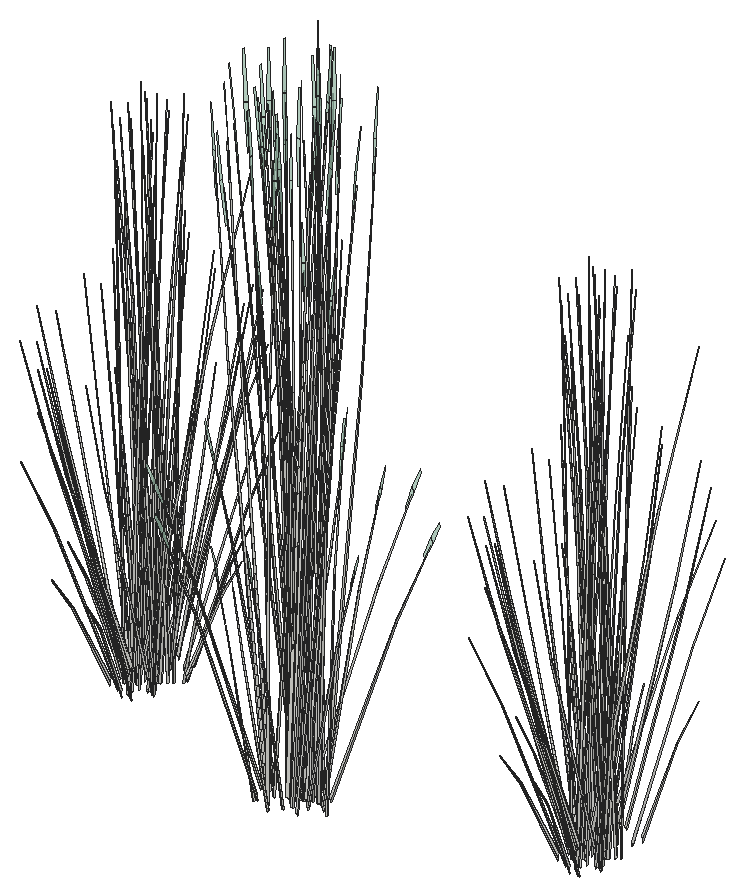
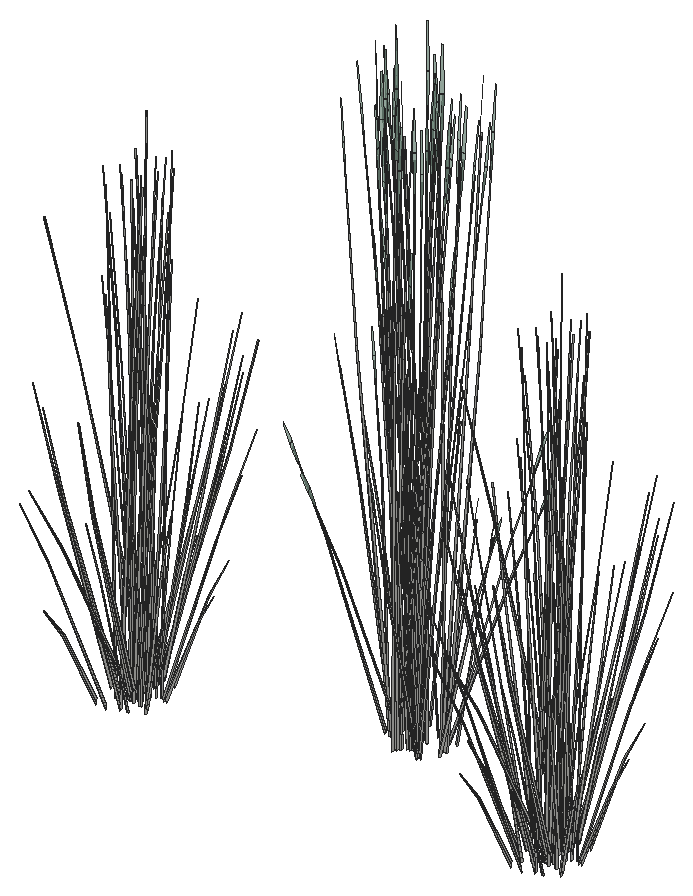
# SketchUp Ruby script. Lengths in inches.
U = 1.inch
M = Sketchup.active_model
def pt(a) = Geom::Point3d.new(a.map { |v| v * U })
def face(e, loops, mat)
  f = e.add_face(loops[0].map { |a| pt(a) })
  loops[1..].each { |l| e.add_face(l.map { |a| pt(a) }).erase! }
  f.material = f.back_material = mat if mat
  f
end
# faces: each face lists its corners as indices into pts; further lists are holes
def faces(e, pts, list, mat = nil) = list.each { |f| face(e, (f[0].is_a?(Array) ? f : [f]).map { |l| l.map { |i| pts[i] } }, mat) }
# xy, xz, yz: faces in a plane at the given z, y or x. An outline is a flat list of corners, or four numbers for a rectangle; further outlines are holes
def ring(l) = l.size == 4 ? [[l[0], l[1]], [l[2], l[1]], [l[2], l[3]], [l[0], l[3]]] : l.each_slice(2).to_a
def flat(e, list, mat, &to3) = list.each { |f| face(e, (f[0].is_a?(Array) ? f : [f]).map { |l| ring(l).map { |u, v| to3.(u, v) } }, mat) }
def xy(e, z, list, mat = nil) = flat(e, list, mat) { |x, y| [x, y, z] }
def xz(e, y, list, mat = nil) = flat(e, list, mat) { |x, z| [x, y, z] }
def yz(e, x, list, mat = nil) = flat(e, list, mat) { |y, z| [x, y, z] }
def lines(e, pts, list) = list.each { |a, b| e.add_line(pt(pts[a]), pt(pts[b])) }
# prism: a flat outline (further loops are holes) pulled along v
def prism(e, loops, v, mat = nil)
  f = face(e, loops, mat); d = Geom::Vector3d.new(v.map { |x| x * U })
  f.pushpull(f.normal.samedirection?(d) ? d.length : -d.length)
end
def box(e, o, s, mat = nil) = prism(e, [[o, [o[0] + s[0], o[1], o[2]], [o[0] + s[0], o[1] + s[1], o[2]], [o[0], o[1] + s[1], o[2]]]], [0, 0, s[2]], mat)
def at(x, y, z, deg = 0) = Geom::Transformation.translation(pt([x, y, z])) * Geom::Transformation.rotation(ORIGIN, Z_AXIS, deg.degrees)
def axes(o, x, y, z) = Geom::Transformation.new([*x, 0, *y, 0, *z, 0, *pt(o).to_a, 1])
def part(name) = M.definitions.add(name)
# library, detail: a bought-in or finely detailed component or shape, given as its bounding box
def library(name, o, s) = part(name).tap { |d| box(d.entities, o, s) }
def detail(e, o, s) = box(e.add_group.entities, o, s)
def put(e, d, t, mat = nil) = e.add_instance(d, t).tap { |i| i.material = mat if mat }
def group(e, t, mat = nil) = e.add_group.tap { |g| g.transformation = t; g.material = mat if mat }.entities
root = M.entities
M.materials.add("LightPink_Translucent").color = [175, 214, 192]
M.materials["LightPink_Translucent"].alpha = 0.75
c1 = part("blade")
p = [[2.15,0.21,22],[0,0.17,0],[0.09,0.45,0],[2.18,0.31,22],[2.29,0.31,22],[0.38,0.45,0],
  [2.48,0.24,33],[2.49,0.24,33],[2.48,0.22,33]]
faces(c1.entities,p,[[0,1,2,3],[4,5,2,3],[6,3,4,7],[8,0,3,6]])
c2 = part("blade with seeds\#1")
put(c2.entities,c1,at(0,0,0))
c3 = part("seeds")
p = [[0.3,-0.1,1.38],[-0.01,-0.03,1.59],[-0.01,-0.03,0.03],[0.14,-0.07,-0.07],[0.29,-0.03,3],[0.15,0.01,3.11]]
faces(c3.entities,p,[[0,1,2,3],[1,0,4,5]],"LightPink_Translucent")
c4 = part("blade with seeds")
put(c4.entities,c1,at(0,0,0))
put(c4.entities,c3,axes([2.4,0.25,30.99],[1.5799,-0.05474,1.17369],[-0.12525,1.92788,0.29478],[-0.07173,-0.02425,1.56792]))
put(root,c2,axes([371.35,242.3,138.84],[0.07713,0.14131,1.17311],[-0.13499,0.4232,-0.25229],[-0.16789,-0.07845,0.50157]))
put(root,c2,axes([371.62,242.95,140.8],[-0.30983,0.23727,-0.58282],[-0.17267,-0.48842,0.07033],[-0.1497,0.05548,0.82446]))
put(root,c2,axes([371.21,244.49,138.84],[0.12465,0.0301,1.17311],[0.10435,0.44009,-0.25229],[-0.16111,0.10287,0.50157]))
put(root,c2,axes([371.92,241.96,140.8],[-0.35246,-0.01294,-0.58282],[0.02367,-0.54471,0.07033],[-0.14932,-0.05748,0.82446]))
put(root,c2,axes([370.74,242.82,138.99],[0.2222,-0.06377,0.94226],[-0.12306,0.35378,0.69231],[-0.11377,-0.03807,0.20754]))
put(root,c2,axes([371.56,243.125,140.56],[-0.09552,0.48869,-0.41919],[-0.3275,-0.16751,-0.3247],[-0.13186,0.04481,0.80208]))
put(root,c2,axes([371.81,242.07,140.56],[-0.25603,0.35588,-0.41919],[-0.22422,-0.37594,-0.3247],[-0.13008,-0.05415,0.80208]))
put(root,c2,axes([371.01,244.64,138.99],[0.13262,-0.25932,0.94226],[0.07972,0.37767,0.69231],[-0.10192,0.08081,0.20754]))
put(root,c2,axes([371.71,244.02,140.8],[-0.18418,0.4239,-0.58282],[-0.32274,-0.30126,0.07033],[-0.10997,0.15358,0.82446]))
put(root,c2,axes([371.72,244.21,140.56],[0.09058,0.49056,-0.41919],[-0.34303,0.08581,-0.3247],[-0.0983,0.13176,0.80208]))
put(root,c2,axes([372.4,241.33,140.56],[-0.34793,0.12771,-0.41919],[-0.06086,-0.48364,-0.3247],[-0.09345,-0.1386,0.80208]))
put(root,c2,axes([372.54,241.32,140.8],[-0.30066,-0.25968,-0.58282],[0.21367,-0.45504,0.07033],[-0.10893,-0.15505,0.82446]))
put(root,c2,axes([372.26,240.94,138.84],[-0.01129,0.1776,1.17311],[-0.30276,0.18194,-0.25229],[-0.08565,-0.21818,0.50157]))
put(root,c2,axes([371.7,240.74,138.99],[0.19397,0.16559,0.94226],[-0.26061,0.14233,0.69231],[-0.0653,-0.13676,0.20754]))
put(root,c2,axes([372.26,245.28,138.84],[0.10609,-0.09706,1.17311],[0.28837,0.22366,-0.25229],[-0.06892,0.22965,0.50157]))
put(root,c2,axes([372.16,244.88,140.8],[-0.00917,0.49695,-0.58282],[-0.38634,-0.03338,0.07033],[-0.04077,0.21053,0.82446]))
put(root,c2,axes([372.24,245.05,140.56],[0.25241,0.36098,-0.41919],[-0.26664,0.31614,-0.3247],[-0.0384,0.18341,0.80208]))
put(root,c2,axes([373.06,243.43,138.71],[0.18468,-0.56014,0.19741],[0.38374,0.26958,0.41019],[-0.08846,0,1.31701]))
put(root,c2,axes([372.58,245.86,138.99],[-0.02727,-0.31739,0.94226],[0.24024,0.20133,0.69231],[-0.03604,0.15684,0.20754]))
put(root,c2,axes([372.8,243.62,138.95],[0.02352,0.53984,0.36702],[-0.39046,0.04882,-0.17663],[-0.03957,-0.09664,1.17838]))
put(root,c2,axes([373.08,245.01,138.75],[0.38104,0,0.40731],[0,0.5562,0],[-0.08679,0,1.29208]))
put(root,c2,axes([372.94,243.63,138.65],[0.42608,-0.21614,0.37535],[0.14817,0.61757,0.14729],[-0.07829,-0.00755,1.30318]))
put(root,c2,axes([373.17,241.11,140.56],[-0.34661,-0.13468,-0.41919],[0.1188,-0.46175,-0.3247],[-0.03178,-0.18591,0.80208]))
put(root,c2,axes([371.96,242.1,138.75],[-0.19052,0.46527,0.40731],[-0.34163,-0.2781,0],[0.04339,-0.10597,1.29208]))
put(root,c2,axes([373.28,243.74,138.95],[0.34335,0.2412,0.36702],[-0.16524,0.50118,-0.17663],[-0.07915,0,1.17838]))
put(root,c2,axes([372.7,243.15,138.65],[0.3458,0.41219,0.37535],[-0.30525,0.4897,0.14729],[-0.03451,-0.09937,1.30318]))
put(root,c2,axes([372.13,243.87,138.75],[0.37869,0.14361,0.14473],[-0.10717,0.52552,0.28783],[-0.00184,-0.09078,1.3159]))
put(root,c2,axes([373.3,241.19,140.8],[-0.16829,-0.43684,-0.58282],[0.34641,-0.24345,0.07033],[-0.03935,-0.21107,0.82446]))
put(root,c2,axes([372.55,242.77,138.86],[-0.34006,-0.0959,0.11878],[0.05903,-0.46856,-0.33919],[0.03492,-0.08527,1.03975]))
put(root,c2,axes([372.64,242.97,138.95],[-0.31983,0.29864,0.36702],[-0.22522,-0.45236,-0.17663],[0.03957,-0.09664,1.17838]))
put(root,c2,axes([373.36,243.58,138.65],[0.08028,-0.62833,0.37535],[0.45342,0.12787,0.14729],[-0.04378,0.09182,1.30318]))
put(root,c2,axes([372.15,242.28,138.75],[0.10113,0.5342,0.14473],[-0.37638,0.13191,0.28783],[0.05484,-0.04764,1.3159]))
put(root,c2,axes([374.08,243.92,138.75],[-0.10113,-0.5342,0.14473],[0.37638,-0.13191,0.28783],[-0.05484,0.04764,1.3159]))
put(root,c2,axes([372.875,242.61,138.67],[-0.08028,0.62833,0.4036],[-0.45342,-0.12787,0.15838],[0.04378,-0.09182,1.40127]))
put(root,c2,axes([373.68,243.43,138.86],[0.34006,0.0959,0.11878],[-0.05903,0.46856,-0.33919],[-0.03492,0.08527,1.03975]))
put(root,c2,axes([373.14,241.51,138.75],[-0.27756,0.39059,0.14473],[-0.26921,-0.39362,0.28783],[0.05668,0.04314,1.3159]))
put(root,c2,axes([372.78,244.42,139.46],[-0.05512,-0.14131,1.45254],[0.38487,-0.04873,0.11368],[0.05107,0.30608,0.51915]))
put(root,c2,axes([373.39,239.95,138.99],[0.06291,0.30716,0.94226],[-0.25998,-0.14458,0.69231],[0.01779,-0.16295,0.20754]))
put(root,c2,axes([374.1,242.33,138.75],[-0.37869,-0.14361,0.14473],[0.10717,-0.52552,0.28783],[0.00184,0.09078,1.3159]))
put(root,c2,axes([372.96,242.45,138.95],[-0.34335,-0.2412,0.36702],[0.16524,-0.50118,-0.17663],[0.07915,0,1.17838]))
put(root,c2,axes([374.27,244.09,138.75],[0.19052,-0.46527,0.40731],[0.34163,0.2781,0],[-0.04339,0.10597,1.29208]))
put(root,c2,axes([372.99,245.4,140.56],[0.34661,0.13468,-0.41919],[-0.1188,0.46175,-0.3247],[0.03178,0.18591,0.80208]))
put(root,c2,axes([373.15,241.1875,138.75],[-0.38104,0,0.40731],[0,-0.5562,0],[0.08679,0,1.29208]))
put(root,c2,axes([373.03,242.24,138.86],[-0.11112,-0.46318,0.11878],[0.31732,-0.1622,-0.33919],[0.06984,0,1.03975]))
put(root,c2,axes([373.43,242.58,138.95],[-0.02352,-0.53984,0.36702],[0.39046,-0.04882,-0.17663],[0.03957,0.09664,1.17838]))
put(root,c2,axes([373.81,240.52,138.84],[-0.09372,0.11973,1.17311],[-0.31002,-0.15578,-0.25229],[0.042,-0.24224,0.50157]))
put(root,c2,axes([373.6,242.57,138.86],[0.22894,-0.36728,0.11878],[0.25829,0.30636,-0.33919],[0.03492,0.08527,1.03975]))
put(root,c2,axes([374,241.62,140.8],[0.00917,-0.49695,-0.58282],[0.38634,0.03338,0.07033],[0.04077,-0.21053,0.82446]))
put(root,c2,axes([374.31,242.18,138.75],[-0.19052,-0.46527,0.40731],[0.34163,-0.2781,0],[0.04339,0.10597,1.29208]))
put(root,c2,axes([373.8,245.95,138.84],[0.03128,-0.17277,1.17311],[0.3195,-0.11135,-0.25229],[0.05981,0.23468,0.50157]))
put(root,c2,axes([374.47,246.31,138.99],[-0.1727,-0.20718,0.94226],[0.27339,-0.08175,0.69231],[0.04895,0.14972,0.20754]))
put(root,c2,axes([374.29,241.65,138.99],[-0.10956,0.27991,0.94226],[-0.11132,-0.36143,0.69231],[0.0943,-0.09749,0.20754]))
put(root,c2,axes([373.76,245.17,140.56],[0.34793,-0.12771,-0.41919],[0.06086,0.48364,-0.3247],[0.09345,0.1386,0.80208]))
put(root,c2,axes([373.06,242.34,139.05],[-0.35877,0.01358,1.15892],[0.093,-0.61462,0.4907],[0.19631,0.14537,1.09393]))
put(root,c2,axes([374.44,242.29,140.56],[-0.09058,-0.49056,-0.41919],[0.34303,-0.08581,-0.3247],[0.0983,-0.13176,0.80208]))
put(root,c2,axes([374.79,241.61,138.91],[-0.01195,0.31879,0.86186],[-0.25381,-0.21053,0.47585],[0.09017,-0.12594,0.67605]))
put(root,c2,axes([374.17,242.65,138.84],[-0.12631,-0.00877,1.17311],[-0.14109,-0.41923,-0.25229],[0.15118,-0.12942,0.50157]))
put(root,c2,axes([375.23,244.55,138.99],[-0.22657,0.01287,0.94226],[0.1616,-0.32149,0.69231],[0.10799,0.06323,0.20754]))
put(root,c2,axes([374.35,244.43,140.82],[0.25603,-0.35588,-0.4653],[0.22422,0.37594,-0.36041],[0.13008,0.05415,0.89031]))
put(root,c2,axes([374.6,243.375,140.56],[0.09552,-0.48869,-0.41919],[0.3275,0.16751,-0.3247],[0.13186,-0.04481,0.80208]))
put(root,c2,axes([374.74,244.82,139.03],[-0.06748,-0.45162,0.05338],[0.27185,-0.10383,-0.708],[0.13761,0.02863,0.63462]))
put(root,c2,axes([374.24,244.54,141.1],[0.35246,0.01294,-0.64693],[-0.02367,0.54471,0.07807],[0.14932,0.05748,0.91515]))
put(root,c2,axes([374.54,243.55,140.8],[0.30983,-0.23727,-0.58282],[0.17267,0.48842,0.07033],[0.1497,-0.05548,0.82446]))
put(root,c2,axes([375.03,244.93,138.84],[-0.06011,-0.15688,1.17311],[0.18125,-0.38733,-0.25229],[0.15683,0.11528,0.50157]))
put(root,c4,axes([388.22,237.2,139.53],[0.1661,0.03656,1.30132],[0.10705,0.37341,-0.27986],[-0.22562,0.0699,0.55638]))
put(root,c4,axes([388.86,235.39,139.53],[0.09331,0.12399,1.30132],[-0.21502,0.33702,-0.27986],[-0.22079,-0.08055,0.55638]))
put(root,c4,axes([389.75,237.98,139.33],[-0.29882,0.44625,0],[-0.49993,-0.24886,-0.46963],[-0.11386,-0.05668,1.48977]))
put(root,c4,axes([389.2,238.63,139.53],[0.15082,-0.07025,1.30132],[0.37238,0.21183,-0.27986],[-0.11083,0.18329,0.55638]))
put(root,c4,axes([388.99,234.62,139.11],[-0.13787,0.36364,-0.03542],[-0.42434,-0.11186,-0.16061],[-0.06443,-0.05948,0.52975]))
put(root,c4,axes([389.625,234.16,139.53],[-0.02894,0.14568,1.30132],[-0.4231,0.12195,-0.27986],[-0.0989,-0.1883,0.55638]))
put(root,c4,axes([388.76,236.28,139.33],[-0.59763,0,0],[0,-0.49772,-0.46963],[0,-0.11336,1.48977]))
put(root,c4,axes([389.22,236.15,139.29],[-0.44456,0.37441,0.27988],[-0.44483,-0.37047,-0.33208],[-0.01552,-0.10632,1.50045]))
put(root,c4,axes([391.23,237.0625,139.41],[-0.4667,-0.35844,-0.22925],[0.39271,-0.40249,0.50168],[-0.12567,0.04193,1.53076]))
put(root,c4,axes([390.01,237.75,139.43],[0.44731,0.22267,0.45182],[-0.26736,0.39927,0],[-0.10188,-0.05071,1.43328]))
put(root,c4,axes([390.43,236.93,139.39],[0.12668,-0.5277,-0.2132],[0.60063,0.09198,0.46656],[-0.10495,-0.07287,1.42361]))
put(root,c4,axes([390.65,237.06,139.55],[-0.0922,0.39744,0.13176],[-0.45047,-0.06899,-0.37626],[-0.08198,-0.04081,1.15337]))
put(root,c4,axes([389.125,236.36,139.43],[0,0.44533,0.45182],[-0.53472,0,0],[0,-0.10143,1.43328]))
put(root,c4,axes([391.57,238.04,139.17],[-0.29509,-0.44781,-0.04679],[0.49993,-0.24886,0.46963],[-0.12319,0.04264,1.48904]))
put(root,c4,axes([389.31,238.29,139.74],[0.43418,-0.07886,0.05922],[0.09982,0.31771,-0.78537],[-0.02753,0.16083,0.70398]))
put(root,c4,axes([390.63,234.16,139.11],[-0.33028,0.25548,-0.03542],[-0.30262,-0.27981,-0.16061],[-0.02131,-0.07928,0.52975]))
put(root,c4,axes([390.5,236.68,139.32],[0.60408,0.09383,0.41637],[-0.12294,0.52992,0.16339],[-0.08828,-0.05117,1.44559]))
put(root,c4,axes([390.17,237.52,139.42],[0.51358,-0.1182,0.16054],[0.12682,0.43988,0.31929],[-0.0458,-0.06409,1.4597]))
put(root,c4,axes([390.83,237.59,139.17],[-0.48183,-0.19993,0],[0.23189,-0.41543,0],[0,0,1.48063]))
put(root,c4,axes([391.95,238.09,139.33],[0.29882,0.44625,0],[-0.49993,0.24886,-0.46963],[-0.11386,0.05668,1.48977]))
put(root,c4,axes([391.7,237.55,139.42],[0.13807,-0.44258,0.16054],[0.50524,0.12525,0.31929],[-0.08728,0.00216,1.4597]))
put(root,c4,axes([391.47,236.96,139.55],[0.3531,0.26757,0.13176],[-0.29453,0.30187,-0.37626],[-0.08198,0.04081,1.15337]))
put(root,c4,axes([391.34,236.63,139.26],[-0.44456,-0.3833,-0.05579],[0.44483,-0.38354,0],[-0.01552,-0.01339,1.5977]))
put(root,c4,axes([391.59,237.8125,139.29],[0.59835,0.14475,0.27988],[-0.14969,0.51739,-0.33208],[-0.09903,0.06475,1.50045]))
put(root,c4,axes([391.84,237.78,139.43],[0.44731,-0.22267,0.45182],[0.26736,0.39927,0],[-0.10188,0.05071,1.43328]))
put(root,c4,axes([390.45,236.1875,139.32],[0.2078,0.49797,0.41637],[-0.59373,0.17316,0.16339],[0.00726,-0.0915,1.44559]))
put(root,c4,axes([390.94,237.42,139.18],[-0.15594,-0.38394,0],[0.4453,-0.13445,0],[0,0,1.40478]))
put(root,c4,axes([392.49,236.42,139.42],[-0.37551,-0.32439,0.16054],[0.37842,-0.31463,0.31929],[-0.04147,0.06625,1.4597]))
put(root,c4,axes([391.19,236.23,139.18],[0,-0.51528,0],[0.59763,0,0],[0,0,1.63305]))
put(root,c4,axes([390.64,236.32,139.38],[0.53851,0.21584,0.21899],[-0.25917,0.44849,0.45502],[0,-0.10338,1.46094]))
put(root,c4,axes([391.49,236.4375,139.26],[0,0.51503,-0.0513],[-0.59763,0,0],[0,0.01619,1.63225]))
put(root,c4,axes([390.22,235.24,139.42],[-0.13807,0.44258,0.16054],[-0.50524,-0.12525,0.31929],[0.08728,-0.00216,1.4597]))
put(root,c4,axes([391.21,237.43,139.25],[0.2078,0.51161,-0.05471],[-0.59373,0.17927,0],[0.00726,0.01787,1.56677]))
put(root,c4,axes([389.98,234.69,139.33],[-0.29882,-0.44625,0],[0.49993,-0.24886,-0.46963],[0.11386,-0.05668,1.48977]))
put(root,c4,axes([392.92,236.76,139.17],[-0.59734,-0.00356,-0.04529],[0,-0.49772,0.45448],[-0.01877,0.1133,1.441]))
put(root,c4,axes([391.75,235.26,139.42],[-0.51358,0.1182,0.16054],[-0.12682,-0.43988,0.31929],[0.0458,0.06409,1.4597]))
put(root,c4,axes([390.91,235.91,139.32],[-0.39628,0.40415,0.41637],[-0.4708,-0.35675,0.16339],[0.09554,-0.04033,1.44559]))
put(root,c4,axes([391.59,236.54,139.19],[0.33362,0.28765,0],[-0.33362,0.28765,0],[0,0,1.54032]))
put(root,c4,axes([391.38,237.6,139.18],[0.48183,0.19993,0],[-0.23189,0.41543,0],[0,0,1.59208]))
put(root,c4,axes([391.43,236.11,139.34],[-0.60408,-0.09383,0.44771],[0.12294,-0.52992,0.17569],[0.08828,0.05117,1.5544]))
put(root,c4,axes([391.6,236.35,139.18],[0.53472,0,0],[0,0.46104,0],[0,0,1.6235]))
put(root,c4,axes([391.78,236.3,139.55],[0.4453,-0.12987,0.13176],[0.15594,0.37086,-0.37626],[0,0.08162,1.15337]))
put(root,c4,axes([391.73,234.33,139.53],[-0.13585,0.09014,1.30132],[-0.40687,-0.15777,-0.27986],[0.07542,-0.19621,0.55638]))
put(root,c4,axes([392.8,236.43,139.43],[0,-0.44533,0.45182],[0.53472,0,0],[0,0.10143,1.43328]))
put(root,c4,axes([391.28,235.73,139.55],[0.0922,-0.39744,0.13176],[0.45047,0.06899,-0.37626],[0.08198,0.04081,1.15337]))
put(root,c4,axes([391.92,235.04,139.43],[-0.44731,-0.22267,0.45182],[0.26736,-0.39927,0],[0.10188,0.05071,1.43328]))
put(root,c4,axes([391.53,237.37,139.16],[0.50177,-0.1511,-0.1747],[0.17632,0.43526,0.00007],[0.05539,-0.0167,1.58246]))
put(root,c4,axes([391.39,237.63,139.53],[0.00843,-0.14762,1.30132],[0.40305,-0.1649,-0.27986],[0.12442,0.17669,0.55638]))
put(root,c4,axes([393.16,236.51,139.33],[0.59763,0,0],[0,0.49772,-0.46963],[0,0.11336,1.48977]))
put(root,c4,axes([392.18,234.81,139.33],[0.29882,-0.44625,0],[0.49993,0.24886,-0.46963],[0.11386,0.05668,1.48977]))
put(root,c4,axes([393.91,236.19,139.23],[-0.29631,-0.28477,-0.05904],[0.32453,-0.26092,-0.26768],[0.09195,-0.01837,0.88292]))
put(root,c4,axes([393.04,235.39,139.53],[-0.17074,-0.01319,1.30132],[-0.17492,-0.35385,-0.27986],[0.20976,-0.1001,0.55638]))
put(root,c4,axes([393.35,236.57,138.97],[-0.30783,0.05344,1.28841],[-0.049,-0.4254,0.07375],[0.2156,-0.06439,0.73315]))
put(root,c4,axes([393.4375,237.2,139.53],[-0.1151,-0.10953,1.30132],[0.14976,-0.36232,-0.27986],[0.23288,0.04908,0.55638]))
put(root,c2,axes([409.55,242.3,138.84],[0.07713,0.14131,1.17311],[-0.13499,0.4232,-0.25229],[-0.16789,-0.07845,0.50157]))
put(root,c2,axes([409.82,242.95,140.8],[-0.30983,0.23727,-0.58282],[-0.17267,-0.48842,0.07033],[-0.1497,0.05548,0.82446]))
put(root,c2,axes([409.4,244.49,138.84],[0.12465,0.0301,1.17311],[0.10435,0.44009,-0.25229],[-0.16111,0.10287,0.50157]))
put(root,c2,axes([410.12,241.96,140.8],[-0.35246,-0.01294,-0.58282],[0.02367,-0.54471,0.07033],[-0.14932,-0.05748,0.82446]))
put(root,c2,axes([408.93,242.82,138.99],[0.2222,-0.06377,0.94226],[-0.12306,0.35378,0.69231],[-0.11377,-0.03807,0.20754]))
put(root,c2,axes([409.75,243.125,140.56],[-0.09552,0.48869,-0.41919],[-0.3275,-0.16751,-0.3247],[-0.13186,0.04481,0.80208]))
put(root,c2,axes([410,242.07,140.56],[-0.25603,0.35588,-0.41919],[-0.22422,-0.37594,-0.3247],[-0.13008,-0.05415,0.80208]))
put(root,c2,axes([409.2,244.64,138.99],[0.13262,-0.25932,0.94226],[0.07972,0.37767,0.69231],[-0.10192,0.08081,0.20754]))
put(root,c2,axes([409.9,244.02,140.8],[-0.18418,0.4239,-0.58282],[-0.32274,-0.30126,0.07033],[-0.10997,0.15358,0.82446]))
put(root,c2,axes([409.91,244.21,140.56],[0.09058,0.49056,-0.41919],[-0.34303,0.08581,-0.3247],[-0.0983,0.13176,0.80208]))
put(root,c2,axes([410.59,241.33,140.56],[-0.34793,0.12771,-0.41919],[-0.06086,-0.48364,-0.3247],[-0.09345,-0.1386,0.80208]))
put(root,c2,axes([410.73,241.32,140.8],[-0.30066,-0.25968,-0.58282],[0.21367,-0.45504,0.07033],[-0.10893,-0.15505,0.82446]))
put(root,c2,axes([410.46,240.94,138.84],[-0.01129,0.1776,1.17311],[-0.30276,0.18194,-0.25229],[-0.08565,-0.21818,0.50157]))
put(root,c2,axes([409.9,240.74,138.99],[0.19397,0.16559,0.94226],[-0.26061,0.14233,0.69231],[-0.0653,-0.13676,0.20754]))
put(root,c2,axes([410.45,245.28,138.84],[0.10609,-0.09706,1.17311],[0.28837,0.22366,-0.25229],[-0.06892,0.22965,0.50157]))
put(root,c2,axes([410.36,244.88,140.8],[-0.00917,0.49695,-0.58282],[-0.38634,-0.03338,0.07033],[-0.04077,0.21053,0.82446]))
put(root,c2,axes([410.4375,245.05,140.56],[0.25241,0.36098,-0.41919],[-0.26664,0.31614,-0.3247],[-0.0384,0.18341,0.80208]))
put(root,c2,axes([411.25,243.43,138.71],[0.18468,-0.56014,0.19741],[0.38374,0.26958,0.41019],[-0.08846,0,1.31701]))
put(root,c2,axes([410.77,245.86,138.99],[-0.02727,-0.31739,0.94226],[0.24024,0.20133,0.69231],[-0.03604,0.15684,0.20754]))
put(root,c2,axes([410.99,243.62,138.95],[0.02352,0.53984,0.36702],[-0.39046,0.04882,-0.17663],[-0.03957,-0.09664,1.17838]))
put(root,c2,axes([411.28,245.01,138.75],[0.38104,0,0.40731],[0,0.5562,0],[-0.08679,0,1.29208]))
put(root,c2,axes([411.13,243.63,138.65],[0.42608,-0.21614,0.37535],[0.14817,0.61757,0.14729],[-0.07829,-0.00755,1.30318]))
put(root,c2,axes([411.36,241.11,140.56],[-0.34661,-0.13468,-0.41919],[0.1188,-0.46175,-0.3247],[-0.03178,-0.18591,0.80208]))
put(root,c2,axes([410.15,242.1,138.75],[-0.19052,0.46527,0.40731],[-0.34163,-0.2781,0],[0.04339,-0.10597,1.29208]))
put(root,c2,axes([411.47,243.74,138.95],[0.34335,0.2412,0.36702],[-0.16524,0.50118,-0.17663],[-0.07915,0,1.17838]))
put(root,c2,axes([410.89,243.15,138.65],[0.3458,0.41219,0.37535],[-0.30525,0.4897,0.14729],[-0.03451,-0.09937,1.30318]))
put(root,c2,axes([410.32,243.87,138.75],[0.37869,0.14361,0.14473],[-0.10717,0.52552,0.28783],[-0.00184,-0.09078,1.3159]))
put(root,c2,axes([411.49,241.19,140.8],[-0.16829,-0.43684,-0.58282],[0.34641,-0.24345,0.07033],[-0.03935,-0.21107,0.82446]))
put(root,c2,axes([410.74,242.77,138.86],[-0.34006,-0.0959,0.11878],[0.05903,-0.46856,-0.33919],[0.03492,-0.08527,1.03975]))
put(root,c2,axes([410.83,242.97,138.95],[-0.31983,0.29864,0.36702],[-0.22522,-0.45236,-0.17663],[0.03957,-0.09664,1.17838]))
put(root,c2,axes([411.55,243.58,138.65],[0.08028,-0.62833,0.37535],[0.45342,0.12787,0.14729],[-0.04378,0.09182,1.30318]))
put(root,c2,axes([410.34,242.28,138.75],[0.10113,0.5342,0.14473],[-0.37638,0.13191,0.28783],[0.05484,-0.04764,1.3159]))
put(root,c2,axes([412.28,243.92,138.75],[-0.10113,-0.5342,0.14473],[0.37638,-0.13191,0.28783],[-0.05484,0.04764,1.3159]))
put(root,c2,axes([411.07,242.61,138.67],[-0.08028,0.62833,0.4036],[-0.45342,-0.12787,0.15838],[0.04378,-0.09182,1.40127]))
put(root,c2,axes([411.875,243.43,138.86],[0.34006,0.0959,0.11878],[-0.05903,0.46856,-0.33919],[-0.03492,0.08527,1.03975]))
put(root,c2,axes([411.33,241.51,138.75],[-0.27756,0.39059,0.14473],[-0.26921,-0.39362,0.28783],[0.05668,0.04314,1.3159]))
put(root,c2,axes([410.98,244.42,139.46],[-0.05512,-0.14131,1.45254],[0.38487,-0.04873,0.11368],[0.05107,0.30608,0.51915]))
put(root,c2,axes([411.58,239.95,138.99],[0.06291,0.30716,0.94226],[-0.25998,-0.14458,0.69231],[0.01779,-0.16295,0.20754]))
put(root,c2,axes([412.3,242.33,138.75],[-0.37869,-0.14361,0.14473],[0.10717,-0.52552,0.28783],[0.00184,0.09078,1.3159]))
put(root,c2,axes([411.15,242.45,138.95],[-0.34335,-0.2412,0.36702],[0.16524,-0.50118,-0.17663],[0.07915,0,1.17838]))
put(root,c2,axes([412.47,244.09,138.75],[0.19052,-0.46527,0.40731],[0.34163,0.2781,0],[-0.04339,0.10597,1.29208]))
put(root,c2,axes([411.1875,245.4,140.56],[0.34661,0.13468,-0.41919],[-0.1188,0.46175,-0.3247],[0.03178,0.18591,0.80208]))
put(root,c2,axes([411.34,241.1875,138.75],[-0.38104,0,0.40731],[0,-0.5562,0],[0.08679,0,1.29208]))
put(root,c2,axes([411.23,242.24,138.86],[-0.11112,-0.46318,0.11878],[0.31732,-0.1622,-0.33919],[0.06984,0,1.03975]))
put(root,c2,axes([411.625,242.58,138.95],[-0.02352,-0.53984,0.36702],[0.39046,-0.04882,-0.17663],[0.03957,0.09664,1.17838]))
put(root,c2,axes([412,240.52,138.84],[-0.09372,0.11973,1.17311],[-0.31002,-0.15578,-0.25229],[0.042,-0.24224,0.50157]))
put(root,c2,axes([411.79,242.57,138.86],[0.22894,-0.36728,0.11878],[0.25829,0.30636,-0.33919],[0.03492,0.08527,1.03975]))
put(root,c2,axes([412.19,241.62,140.8],[0.00917,-0.49695,-0.58282],[0.38634,0.03338,0.07033],[0.04077,-0.21053,0.82446]))
put(root,c2,axes([412.5,242.18,138.75],[-0.19052,-0.46527,0.40731],[0.34163,-0.2781,0],[0.04339,0.10597,1.29208]))
put(root,c2,axes([412,245.95,138.84],[0.03128,-0.17277,1.17311],[0.3195,-0.11135,-0.25229],[0.05981,0.23468,0.50157]))
put(root,c2,axes([412.67,246.31,138.99],[-0.1727,-0.20718,0.94226],[0.27339,-0.08175,0.69231],[0.04895,0.14972,0.20754]))
put(root,c2,axes([412.49,241.65,138.99],[-0.10956,0.27991,0.94226],[-0.11132,-0.36143,0.69231],[0.0943,-0.09749,0.20754]))
put(root,c2,axes([411.96,245.17,140.56],[0.34793,-0.12771,-0.41919],[0.06086,0.48364,-0.3247],[0.09345,0.1386,0.80208]))
put(root,c2,axes([411.25,242.34,139.05],[-0.35877,0.01358,1.15892],[0.093,-0.61462,0.4907],[0.19631,0.14537,1.09393]))
put(root,c2,axes([412.64,242.29,140.56],[-0.09058,-0.49056,-0.41919],[0.34303,-0.08581,-0.3247],[0.0983,-0.13176,0.80208]))
put(root,c2,axes([412.98,241.61,138.91],[-0.01195,0.31879,0.86186],[-0.25381,-0.21053,0.47585],[0.09017,-0.12594,0.67605]))
put(root,c2,axes([412.37,242.65,138.84],[-0.12631,-0.00877,1.17311],[-0.14109,-0.41923,-0.25229],[0.15118,-0.12942,0.50157]))
